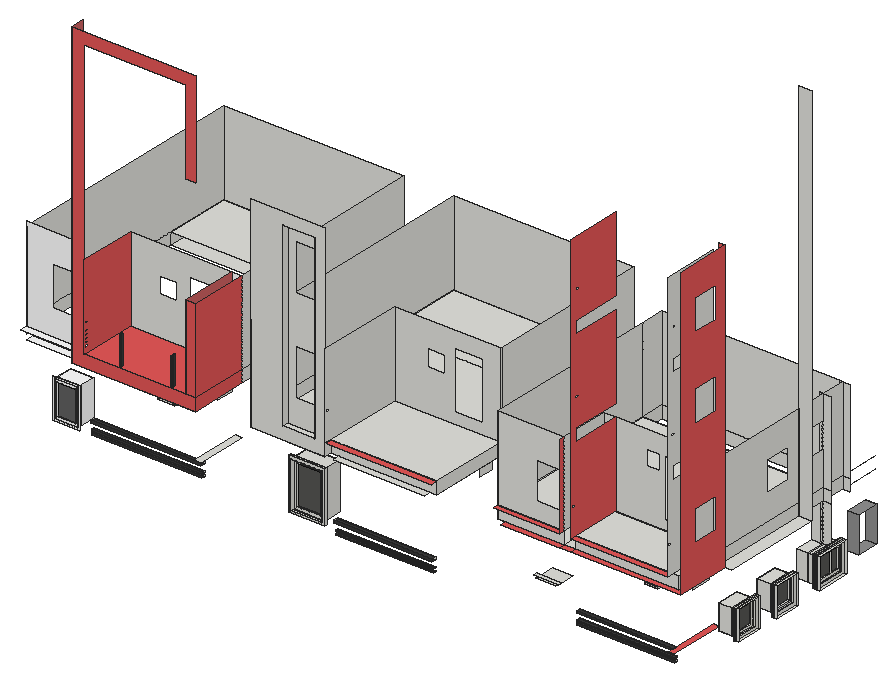
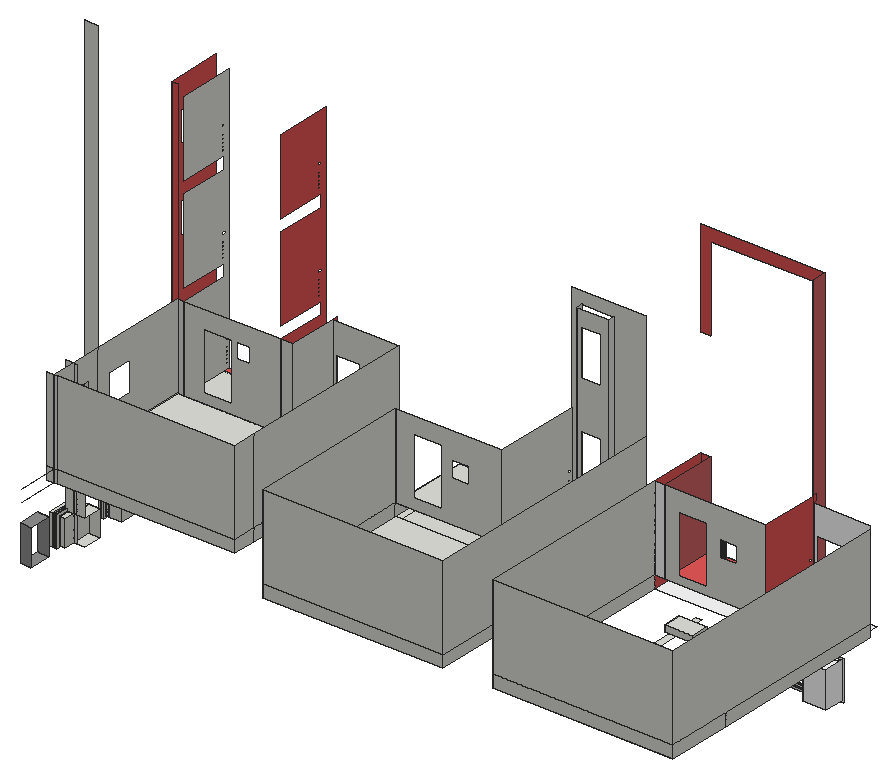
# SketchUp Ruby script. Lengths in inches.
U = 1.inch
M = Sketchup.active_model
def pt(a) = Geom::Point3d.new(a.map { |v| v * U })
def face(e, loops, mat)
  f = e.add_face(loops[0].map { |a| pt(a) })
  loops[1..].each { |l| e.add_face(l.map { |a| pt(a) }).erase! }
  f.material = f.back_material = mat if mat
  f
end
# faces: each face lists its corners as indices into pts; further lists are holes
def faces(e, pts, list, mat = nil) = list.each { |f| face(e, (f[0].is_a?(Array) ? f : [f]).map { |l| l.map { |i| pts[i] } }, mat) }
# xy, xz, yz: faces in a plane at the given z, y or x. An outline is a flat list of corners, or four numbers for a rectangle; further outlines are holes
def ring(l) = l.size == 4 ? [[l[0], l[1]], [l[2], l[1]], [l[2], l[3]], [l[0], l[3]]] : l.each_slice(2).to_a
def flat(e, list, mat, &to3) = list.each { |f| face(e, (f[0].is_a?(Array) ? f : [f]).map { |l| ring(l).map { |u, v| to3.(u, v) } }, mat) }
def xy(e, z, list, mat = nil) = flat(e, list, mat) { |x, y| [x, y, z] }
def xz(e, y, list, mat = nil) = flat(e, list, mat) { |x, z| [x, y, z] }
def yz(e, x, list, mat = nil) = flat(e, list, mat) { |y, z| [x, y, z] }
def lines(e, pts, list) = list.each { |a, b| e.add_line(pt(pts[a]), pt(pts[b])) }
# prism: a flat outline (further loops are holes) pulled along v
def prism(e, loops, v, mat = nil)
  f = face(e, loops, mat); d = Geom::Vector3d.new(v.map { |x| x * U })
  f.pushpull(f.normal.samedirection?(d) ? d.length : -d.length)
end
def box(e, o, s, mat = nil) = prism(e, [[o, [o[0] + s[0], o[1], o[2]], [o[0] + s[0], o[1] + s[1], o[2]], [o[0], o[1] + s[1], o[2]]]], [0, 0, s[2]], mat)
def at(x, y, z, deg = 0) = Geom::Transformation.translation(pt([x, y, z])) * Geom::Transformation.rotation(ORIGIN, Z_AXIS, deg.degrees)
def axes(o, x, y, z) = Geom::Transformation.new([*x, 0, *y, 0, *z, 0, *pt(o).to_a, 1])
def part(name) = M.definitions.add(name)
# library, detail: a bought-in or finely detailed component or shape, given as its bounding box
def library(name, o, s) = part(name).tap { |d| box(d.entities, o, s) }
def detail(e, o, s) = box(e.add_group.entities, o, s)
def put(e, d, t, mat = nil) = e.add_instance(d, t).tap { |i| i.material = mat if mat }
def group(e, t, mat = nil) = e.add_group.tap { |g| g.transformation = t; g.material = mat if mat }.entities
root = M.entities
M.materials.add("Generic").color = [145, 145, 145]
M.materials.add("Generic\#1").color = [206, 99, 99]
M.materials.add("Generic\#2").color = [229, 87, 87]
M.materials.add("[Color M00]").color = [255, 255, 255]
M.materials.add("[Color M07]").color = [58, 58, 58]
M.materials.add("[Translucent Glass Gray]").color = [0, 0, 0]
M.materials["[Translucent Glass Gray]"].alpha = 0.62
M.materials.add("[Translucent Glass Gray]1").color = [128, 128, 128]
M.materials["[Translucent Glass Gray]1"].alpha = 0.5
c1 = part("Group\#5")
xy(c1.entities,0,[[0,0,46.6875,6]],"[Color M00]")
xy(c1.entities,4.48,[[4.48,0,42.2,3]],"[Color M00]")
xy(c1.entities,67.45,[[4.48,0,42.2,3]],"[Color M00]")
xy(c1.entities,71.9375,[[0,0,46.6875,6]],"[Color M00]")
xz(c1.entities,0,[[[0,0,46.6875,71.9375],[4.48,4.48,42.2,67.45]]],"[Color M00]")
xz(c1.entities,3,[[4.48,4.48,42.2,67.45]],"[Translucent Glass Gray]")
xz(c1.entities,6,[[0,0,46.6875,71.9375]],"[Color M00]")
yz(c1.entities,0,[[0,0,6,71.9375]],"[Color M00]")
yz(c1.entities,4.48,[[0,4.48,3,67.45]],"[Color M00]")
yz(c1.entities,42.2,[[0,4.48,3,67.45]],"[Color M00]")
yz(c1.entities,46.6875,[[0,0,6,71.9375]],"[Color M00]")
c2 = part("Group\#9")
xy(c2.entities,0,[[0,0,6,44.5]])
xy(c2.entities,4.64,[[3,4.64,6,39.86]])
xy(c2.entities,45.36,[[3,4.64,6,39.86]])
xy(c2.entities,50,[[0,0,6,44.5]])
xz(c2.entities,0,[[0,0,6,50]])
xz(c2.entities,4.64,[[3,4.64,6,45.36]])
xz(c2.entities,39.86,[[3,4.64,6,45.36]])
xz(c2.entities,44.5,[[0,0,6,50]])
yz(c2.entities,0,[[0,0,44.5,50]])
yz(c2.entities,3,[[4.64,4.64,39.86,45.36]],"[Translucent Glass Gray]")
yz(c2.entities,6,[[[0,0,44.5,50],[4.64,4.64,39.86,45.36]]])
c3 = part("Group\#8")
xy(c3.entities,0,[[0,0,6,59.4375]])
xy(c3.entities,4.64,[[3,4.64,6,54.8]])
xy(c3.entities,46.99,[[3,4.64,6,54.8]])
xy(c3.entities,51.625,[[0,0,6,59.4375]])
xz(c3.entities,0,[[0,0,6,51.625]])
xz(c3.entities,4.64,[[3,4.64,6,46.99]])
xz(c3.entities,54.8,[[3,4.64,6,46.99]])
xz(c3.entities,59.4375,[[0,0,6,51.625]])
yz(c3.entities,0,[[0,0,59.4375,51.625]])
yz(c3.entities,3,[[4.64,4.64,54.8,46.99]],"[Translucent Glass Gray]")
yz(c3.entities,6,[[[0,0,59.4375,51.625],[4.64,4.64,54.8,46.99]]])
c4 = part("Group\#11")
xy(c4.entities,0,[[0,0,27.8125,3]])
xy(c4.entities,27.8125,[[0,0,27.8125,3]])
xz(c4.entities,0,[[0,0,27.8125,27.8125]],"[Translucent Glass Gray]1")
xz(c4.entities,3,[[0,0,27.8125,27.8125]],"[Translucent Glass Gray]1")
yz(c4.entities,0,[[0,0,3,27.8125]])
yz(c4.entities,27.8125,[[0,0,3,27.8125]])
c5 = part("Group\#12")
xy(c5.entities,0,[[0,0,20.25,3]])
xy(c5.entities,24.8125,[[0,0,20.25,3]])
xz(c5.entities,0,[[0,0,20.25,24.8125]],"[Translucent Glass Gray]1")
xz(c5.entities,3,[[0,0,20.25,24.8125]],"[Translucent Glass Gray]1")
yz(c5.entities,0,[[0,0,3,24.8125]])
yz(c5.entities,20.25,[[0,0,3,24.8125]])
xy(root,222.81,[[263.03,103.34,482.8125,108.98]],"[Color M07]")
xy(root,223.99,[[1230.96,102.74,1425.14,108.3]],"[Color M07]")
xy(root,224.3,[[758.59,90.7,954.11,95.51]],"[Color M07]")
xy(root,224.34,[[1452.58,215.23,1457.58,268.54],[1457.58,215.23,1462.21,268.54]])
xy(root,224.91,[[1452.58,310.17,1457.58,363.48],[1457.58,310.17,1462.21,363.48]])
xy(root,226.17,[[758.59,90.7,954.11,95.51]],"[Color M07]")
xy(root,226.18,[[263.03,103.34,482.8125,108.98]],"[Color M07]")
xy(root,226.74,[[1230.96,102.74,1425.14,108.3]],"[Color M07]")
xy(root,227.46,[[1448.58,417.16,1452.58,485.41],[1452.58,417.16,1456.58,485.41],[1456.58,417.16,1462.21,485.41]])
xy(root,228.54,[[192.03,99.8125,238.71,138.75]],"[Color M00]")
xy(root,228.75,[[1419.77,219.63,1452.58,264.13],[1452.58,219.63,1457.58,264.13]])
xy(root,229.28,[[663.18,93.8125,734.35,99.8125]])
xy(root,229.31,[[1419.77,314.57,1452.58,359.07],[1452.58,314.57,1457.58,359.07]])
xy(root,230.06,[[263.03,103.34,482.8125,108.98]],"[Color M07]")
xy(root,230.43,[[1230.96,102.74,1425.14,108.3]],"[Color M07]")
xy(root,230.98,[[758.59,90.7,954.11,95.51]],"[Color M07]")
xy(root,231.86,[[1413.27,421.57,1435.83,459.8125],[1435.83,421.57,1448.58,459.8125],[1448.58,421.57,1452.58,481],[1452.58,421.57,1456.58,481],[1435.83,459.8125,1448.58,481]])
xy(root,232.86,[[758.59,90.7,954.11,95.51]],"[Color M07]")
xy(root,233.18,[[1230.96,102.74,1425.14,108.3]],"[Color M07]")
xy(root,233.43,[[263.03,103.34,482.8125,108.98]],"[Color M07]")
xy(root,233.65,[[667.55,93.8125,729.98,99.8125],[667.55,99.8125,729.98,137.6875]])
xy(root,239.12,[[1429.21,528.77,1451.02,572.96]],"Generic")
xy(root,245.06,[[443.78,103.76,445.34,107.89],[446.53,103.76,448.09,107.89]])
xy(root,245.06,[[[263.03,100.96,482.8125,108.98],[443.78,103.76,445.34,107.89],[446.53,103.76,448.09,107.89]]],"[Color M07]")
xy(root,245.43,[[1230.96,100.55,1425.14,108.3]],"[Color M07]")
xy(root,245.62,[[333.84,103.76,335.4,107.89]])
xy(root,245.73,[[758.59,87.57,954.11,95.51]],"[Color M07]")
xy(root,245.93,[[336.59,103.76,338.15,107.89]])
xy(root,249.99,[[263.03,100.96,482.8125,108.98]],"[Color M07]")
xy(root,250.36,[[1425.14,88,1435.83,199.25]],"Generic\#2")
xy(root,250.36,[[1230.96,100.55,1425.14,108.3]],"[Color M07]")
xy(root,251.17,[[758.59,87.57,954.11,95.51]],"[Color M07]")
xy(root,262.625,[[482.8125,84.5,495.5,187.125]])
xy(root,275.46,[[808.05,253.75,841.375,258.8125]])
xy(root,275.88,[[331.98,182.0625,365.3125,187.125]])
xy(root,278.22,[[810.81,253.75,838.62,258.8125],[810.81,258.8125,838.62,292.8125]])
xy(root,278.6,[[1292.01,194.1875,1317.77,199.25]])
xy(root,278.63,[[334.74,182.0625,362.55,187.125],[334.74,187.125,362.55,221.125]])
xy(root,278.75,[[1419.77,219.63,1452.58,264.13],[1452.58,219.63,1457.58,264.13]])
xy(root,279.31,[[1419.77,314.57,1452.58,359.07],[1452.58,314.57,1457.58,359.07]])
xy(root,281.36,[[1294.76,194.1875,1315.01,199.25],[1294.76,199.25,1315.01,212.4375]])
xy(root,283.15,[[1452.58,215.23,1457.58,268.54],[1457.58,215.23,1462.21,268.54]])
xy(root,283.49,[[1413.27,421.57,1435.83,459.8125],[1435.83,421.57,1448.58,459.8125],[1448.58,421.57,1452.58,481],[1452.58,421.57,1456.58,481],[1435.83,459.8125,1448.58,481]])
xy(root,283.71,[[1452.58,310.17,1457.58,363.48],[1457.58,310.17,1462.21,363.48]])
xy(root,284.75,[[1156.27,93.8125,1196.2,99.8125],[1156.27,99.8125,1196.2,134.3125]])
xy(root,287.89,[[1448.58,417.16,1452.58,485.41],[1452.58,417.16,1456.58,485.41],[1456.58,417.16,1462.21,485.41]])
xy(root,289.12,[[1151.9,93.8125,1200.57,99.8125]])
xy(root,300.48,[[192.03,99.8125,238.71,138.75]],"[Color M00]")
xy(root,306.03,[[810.81,253.75,838.62,258.8125],[810.81,258.8125,838.62,292.8125]])
xy(root,306.17,[[1294.76,194.1875,1315.01,199.25],[1294.76,199.25,1315.01,212.4375]])
xy(root,306.45,[[334.74,182.0625,362.55,187.125],[334.74,187.125,362.55,221.125]])
xy(root,308.79,[[808.05,253.75,841.375,258.8125]])
xy(root,308.93,[[1292.01,194.1875,1317.77,199.25]])
xy(root,309.2,[[331.98,182.0625,365.3125,187.125]])
xy(root,310.62,[[1429.21,528.77,1451.02,572.96]],"Generic")
xy(root,314.12,[[1327.46,199.25,1383.27,240]])
xy(root,321.51,[[856.48,258.8125,912.29,288.3125]])
xy(root,326.71,[[667.55,93.8125,729.98,99.8125],[667.55,99.8125,729.98,137.6875]])
xy(root,327.08,[[392.26,187.125,448.07,220.9375]])
xy(root,331.08,[[663.18,93.8125,734.35,99.8125]])
xy(root,360,[[594.11,86,741.96,99.8125],[758.59,86,940.8,99.8125],[594.11,99.8125,594.11,459.8125,954.11,459.8125,954.11,258.8125,741.96,258.8125,741.96,99.8125],[741.96,99.8125,758.59,258.8125],[758.59,99.8125,940.8,258.8125],
  [940.8,99.8125,954.11,258.8125],[1075.83,99.8125,1075.83,459.8125,1413.27,459.8125,1413.27,199.25,1207.39,199.25,1207.39,99.8125],[1207.39,99.8125,1230.96,199.25],[1413.27,199.25,1435.83,398.12],[1435.83,199.25,1462.21,398.12],
  [1413.27,398.12,1435.83,459.8125],[135.5,459.8125,495.5,590.625],[594.11,459.8125,954.11,590.625]])
xy(root,360,[[1091.08,88,1207.39,99.8125],[1207.39,88,1230.96,99.8125],[1230.96,88,1230.96,99.8125,1435.83,99.8125,1435.83,199.25,1448.83,199.25,1448.83,88],[1230.96,99.8125,1435.83,199.25]],"Generic\#2")
xy(root,360,[[248.28,71.5,248.28,84.5,147.6875,84.5,147.6875,99.8125,263.03,99.8125,263.03,187.125,495.5,187.125,495.5,71.5]],"[Color M00]")
xy(root,373.375,[[135.5,84.5,248.28,99.8125]],"[Color M00]")
xy(root,384,[[339.06,76.97,340.62,80.4375],[341.81,76.97,343.37,80.4375],[442.43,76.97,444,80.4375],[445.18,76.97,446.75,80.4375],[657.35,86,720.59,99.8125],
  [741.96,99.8125,954.11,258.8125],[1075.83,99.8125,1075.83,459.8125,1435.83,459.8125,1435.83,199.25,1207.39,199.25,1207.39,99.8125],[1230.96,99.8125,1423.39,199.25],[1423.39,99.8125,1435.83,199.25],[135.5,459.8125,495.5,590.625],
  [594.11,459.8125,954.11,590.625]])
xy(root,384,[[[272.78,71.5,475.8125,187.125],[445.18,76.97,446.75,80.4375],[442.43,76.97,444,80.4375],[341.81,76.97,343.37,80.4375],[339.06,76.97,340.62,80.4375]],[741.96,86,954.11,99.8125],[1075.83,88,1207.39,99.8125],[1230.96,88,1423.39,99.8125]],"Generic\#2")
xy(root,384,[[475.8125,71.5,495.5,187.125]],"[Color M00]")
xz(root,71.5,[[248.28,360,495.5,360,495.5,384,272.78,384,272.78,936,475.8125,936,475.8125,768,495.5,768,495.5,960,248.28,960],[475.8125,384,495.5,552]],"Generic\#2")
xz(root,76.97,[[339.06,384,340.62,441.31],[341.81,384,343.37,441.31],[442.43,384,444,438.37],[445.18,384,446.75,441.06]],"[Color M07]")
xz(root,80.4375,[[339.06,384,340.62,394.36],[341.81,384,343.37,394.36],[445.18,384,446.75,394.36]])
xz(root,86,[[[594.11,360,741.96,768],[657.35,384,720.59,744]]])
xz(root,87.57,[[758.59,245.73,954.11,251.17]],"[Color M07]")
xz(root,90.7,[[758.59,224.3,954.11,226.17],[758.59,230.98,954.11,232.86]],"[Color M07]")
xz(root,93.8125,[[[663.18,229.28,734.35,331.08],[667.55,233.65,729.98,326.71]]])
xz(root,95.51,[[758.59,224.3,954.11,226.17],[758.59,230.98,954.11,232.86],[758.59,245.73,954.11,251.17]])
xz(root,99.8125,[[[663.18,229.28,734.35,331.08],[667.55,233.65,729.98,326.71]],[741.96,360,954.11,384],[1075.83,360,1207.39,384],[1230.96,360,1435.83,384],[[657.35,384,720.59,744],[672.35,621.05,712.33,713.66],[672.35,433.8,712.33,526.41]],
  [[1075.83,384,1207.39,552],[1151.9,418.07,1200.57,491.43]]])
xz(root,99.8125,[[[188.42,224.94,242.3125,304.08],[192.03,228.54,238.71,300.48]],[[135.5,373.375,248.28,560.8125],[188.42,424.75,242.3125,503.89]]],"[Color M00]")
xz(root,100.55,[[1230.96,245.43,1425.14,250.36]],"[Color M07]")
xz(root,100.96,[[263.03,245.06,482.8125,249.99]],"[Color M07]")
xz(root,102.74,[[1230.96,223.99,1425.14,226.74],[1230.96,230.43,1425.14,233.18]],"[Color M07]")
xz(root,103.34,[[263.03,222.81,482.8125,226.18],[263.03,230.06,482.8125,233.43]],"[Color M07]")
xz(root,108.3,[[1230.96,223.99,1425.14,226.74],[1230.96,230.43,1425.14,233.18],[1230.96,245.43,1425.14,250.36]])
xz(root,108.98,[[263.03,222.81,482.8125,226.18],[263.03,230.06,482.8125,233.43],[263.03,245.06,482.8125,249.99]])
xz(root,137.6875,[[667.55,233.65,729.98,326.71]])
xz(root,138.75,[[192.03,228.54,238.71,300.48]],"[Color M00]")
xz(root,182.0625,[[[331.98,275.88,365.3125,309.2],[334.74,278.63,362.55,306.45]]])
xz(root,187.125,[[[331.98,275.88,365.3125,309.2],[334.74,278.63,362.55,306.45]],[[272.78,384,475.8125,552],[392.26,399.1875,448.07,512.73],[331.98,461.13,365.3125,494.45]]])
xz(root,187.125,[[475.8125,384,495.5,552]],"[Color M00]")
xz(root,194.1875,[[[1292.01,278.6,1317.77,308.93],[1294.76,281.36,1315.01,306.17]]])
xz(root,199.25,[[[1292.01,278.6,1317.77,308.93],[1294.76,281.36,1315.01,306.17]],[1207.39,384,1230.96,552],[[1230.96,384,1423.39,552],[1327.46,403.35,1383.27,516.9],[1292.01,486.72,1317.77,517.05]],[1423.39,384,1435.83,552]])
xz(root,199.25,[[1435.83,360,1448.83,936]],"Generic\#2")
xz(root,212.4375,[[1294.76,281.36,1315.01,306.17]])
xz(root,215.23,[[1452.58,224.34,1457.58,283.15],[1457.58,224.34,1462.21,283.15]])
xz(root,219.63,[[1419.77,228.75,1452.58,278.75],[1452.58,228.75,1457.58,278.75]])
xz(root,220.9375,[[392.26,313.66,448.07,327.08]])
xz(root,221.125,[[334.74,278.63,362.55,306.45]])
xz(root,240,[[1327.46,297.87,1383.27,314.12]])
xz(root,253.75,[[[808.05,275.46,841.375,308.79],[810.81,278.22,838.62,306.03]]])
xz(root,258.8125,[[[808.05,275.46,841.375,308.79],[810.81,278.22,838.62,306.03]],[[741.96,384,954.11,552],[862.05,405.73,917.86,519.27],[808.05,467.09,841.375,500.42]]])
xz(root,264.13,[[1419.77,228.75,1452.58,278.75],[1452.58,228.75,1457.58,278.75]])
xz(root,268.54,[[1452.58,224.34,1457.58,283.15],[1457.58,224.34,1462.21,283.15]])
xz(root,288.3125,[[856.48,307.2,912.29,321.51]])
xz(root,292.8125,[[810.81,278.22,838.62,306.03]])
xz(root,310.17,[[1452.58,224.91,1457.58,283.71],[1457.58,224.91,1462.21,283.71]])
xz(root,314.57,[[1419.77,229.31,1452.58,279.31],[1452.58,229.31,1457.58,279.31]])
xz(root,359.07,[[1419.77,229.31,1452.58,279.31],[1452.58,229.31,1457.58,279.31]])
xz(root,363.48,[[1452.58,224.91,1457.58,283.71],[1457.58,224.91,1462.21,283.71]])
xz(root,398.12,[[1435.83,360,1462.21,1128]])
xz(root,417.16,[[1448.58,227.46,1452.58,287.89],[1452.58,227.46,1456.58,287.89],[1456.58,227.46,1462.21,287.89]])
xz(root,421.57,[[1413.27,231.86,1435.83,283.49],[1435.83,231.86,1448.58,283.49],[1448.58,231.86,1452.58,283.49],[1452.58,231.86,1456.58,283.49]])
xz(root,459.8125,[[1429.21,231.86,1433.58,283.49],[1433.58,231.86,1435.83,283.49],[1435.83,231.86,1451.02,283.49],[1413.27,283.49,1429.21,360],[1429.21,283.49,1433.58,360],
  [1433.58,283.49,1435.83,360],[1435.83,283.49,1451.02,360],[1075.83,360,1429.21,384],[1429.21,360,1433.58,384],[1433.58,360,1435.83,384],
  [1435.83,360,1451.02,384],[1429.21,384,1433.58,552],[1433.58,384,1435.83,552],[1435.83,384,1451.02,552]])
xz(root,481,[[1435.83,231.86,1448.58,283.49],[1448.58,231.86,1452.58,283.49],[1452.58,231.86,1456.58,283.49]])
xz(root,485.41,[[1448.58,227.46,1452.58,287.89],[1452.58,227.46,1456.58,287.89],[1456.58,227.46,1462.21,287.89]])
xz(root,507.75,[[1075.83,360,1429.21,384],[1429.21,360,1435.83,384],[1435.83,360,1451.02,384],[1075.83,384,1429.21,552],[1429.21,384,1435.83,552],
  [1435.83,384,1451.02,552]])
xz(root,528.77,[[1429.21,239.12,1451.02,310.62]],"Generic")
xz(root,572.96,[[1429.21,239.12,1451.02,310.62]],"Generic")
xz(root,590.625,[[135.5,360,495.5,384],[594.11,360,954.11,384],[135.5,384,495.5,552],[594.11,384,954.11,552]])
yz(root,135.5,[[99.8125,360,459.8125,384],[459.8125,360,590.625,384],[99.8125,384,590.625,552]])
yz(root,192.03,[[99.8125,228.54,138.75,300.48]],"[Color M00]")
yz(root,238.71,[[99.8125,228.54,138.75,300.48]],"[Color M00]")
yz(root,248.28,[[71.5,360,71.5,960,99.8125,960,99.8125,576,90.625,576,90.625,560.8125,99.8125,560.8125,99.8125,373.375,84.5,373.375,84.5,360]],"Generic\#1")
yz(root,263.03,[[103.34,222.81,108.98,226.18],[103.34,230.06,108.98,233.43],[100.96,245.06,108.98,249.99]])
yz(root,272.78,[[[71.5,384,77.61,384,77.61,394.36,74.79,394.36,74.79,397.74,80.4375,397.74,80.4375,394.36,77.61,394.36,77.61,384,187.125,384,187.125,552,71.5,552],[72.41,437.31,80.4375,442.24],[74.79,401.61,80.4375,404.99],[74.79,408.18,80.4375,411.55],[74.79,415.24,80.4375,418.62],[74.79,422.31,80.4375,425.68]]],"Generic\#2")
yz(root,331.98,[[182.0625,275.88,187.125,309.2]])
yz(root,334.74,[[182.0625,278.63,187.125,306.45],[187.125,278.63,221.125,306.45]])
yz(root,339.06,[[76.97,384,80.4375,441.31]],"[Color M07]")
yz(root,340.62,[[76.97,384,80.4375,441.31]],"[Color M07]")
yz(root,341.81,[[76.97,384,80.4375,441.31]],"[Color M07]")
yz(root,343.37,[[76.97,384,80.4375,441.31]],"[Color M07]")
yz(root,362.55,[[182.0625,278.63,187.125,306.45],[187.125,278.63,221.125,306.45]])
yz(root,365.3125,[[182.0625,275.88,187.125,309.2]])
yz(root,392.26,[[187.125,313.66,220.9375,327.08]])
yz(root,442.43,[[76.97,384,80.4375,438.37]],"[Color M07]")
yz(root,444,[[76.97,384,80.4375,438.37]],"[Color M07]")
yz(root,445.18,[[76.97,384,80.4375,441.06]],"[Color M07]")
yz(root,446.75,[[76.97,384,80.4375,441.06]],"[Color M07]")
yz(root,448.07,[[187.125,313.66,220.9375,327.08]])
yz(root,475.8125,[[71.5,384,187.125,552]],"Generic\#1")
yz(root,495.5,[[187.125,360,590.625,384],[187.125,384,590.625,552]])
yz(root,495.5,[[71.5,360,187.125,384],[71.5,384,187.125,552]],"Generic\#2")
yz(root,594.11,[[86,360,459.8125,384],[459.8125,360,590.625,384],[86,384,590.625,552]])
yz(root,657.35,[[86,384,99.8125,744]])
yz(root,663.18,[[93.8125,229.28,99.8125,331.08]])
yz(root,667.55,[[93.8125,233.65,99.8125,326.71],[99.8125,233.65,137.6875,326.71]])
yz(root,720.59,[[86,384,99.8125,744]])
yz(root,729.98,[[93.8125,233.65,99.8125,326.71],[99.8125,233.65,137.6875,326.71]])
yz(root,734.35,[[93.8125,229.28,99.8125,331.08]])
yz(root,741.96,[[86,360,99.8125,384],[[86,384,258.8125,552],[87.39,437.85,95.33,443.28],[90.52,395.27,95.33,397.15],[90.27,401.9,95.08,403.77],[90.33,408.77,95.14,410.65],[90.27,416.28,95.08,418.16],[90.39,422.85,95.2,424.72]]])
yz(root,758.59,[[90.7,224.3,95.51,226.17],[90.7,230.98,95.51,232.86],[87.57,245.73,95.51,251.17]])
yz(root,808.05,[[253.75,275.46,258.8125,308.79]])
yz(root,810.81,[[253.75,278.22,258.8125,306.03],[258.8125,278.22,292.8125,306.03]])
yz(root,838.62,[[253.75,278.22,258.8125,306.03],[258.8125,278.22,292.8125,306.03]])
yz(root,841.375,[[253.75,275.46,258.8125,308.79]])
yz(root,856.48,[[258.8125,307.2,288.3125,321.51]])
yz(root,912.29,[[258.8125,307.2,288.3125,321.51]])
yz(root,954.11,[[99.8125,360,260.5,384],[260.5,360,590.625,384],[258.8125,384,260.5,552],[260.5,384,590.625,552]])
yz(root,1075.83,[[99.8125,360,459.8125,384],[459.8125,360,507.75,384],[99.8125,384,459.8125,552],[459.8125,384,507.75,552]])
yz(root,1207.39,[[99.8125,384,199.25,552]])
yz(root,1207.39,[[88,384,99.8125,552]],"Generic\#2")
yz(root,1230.96,[[102.74,223.99,108.3,226.74],[102.74,230.43,108.3,233.18],[100.55,245.43,108.3,250.36]])
yz(root,1230.96,[[[88,384,199.25,384,199.25,552,99.8125,552,99.8125,576,199.25,576,199.25,744,99.8125,744,99.8125,768,199.25,768,199.25,917.875,88,917.875],[96.68,629.37,106.62,634.31],[88.89,437.21,96.64,442.14],[99.8125,821.5625,106.62,826.5],[101.06,778.5,106.62,781.25],[101.06,785.4375,106.62,788.1875],[101.06,792.4375,106.62,795.1875],[101.06,799.6875,106.62,802.4375],[101.06,806.5625,106.62,809.3125],[101.06,614.37,106.62,617.12],[101.06,607.25,106.62,610],[101.06,600.625,106.62,603.375],[101.06,593.5625,106.62,596.3125],[91.08,422.82,96.64,425.57],[91.08,415.32,96.64,418.07],[91.08,408.7,96.64,411.45],[91.08,401.51,96.64,404.26],[91.08,394.51,96.64,397.26],[101.06,586.3125,106.62,589.0625]]],"Generic\#2")
yz(root,1292.01,[[194.1875,278.6,199.25,308.93]])
yz(root,1294.76,[[194.1875,281.36,199.25,306.17],[199.25,281.36,212.4375,306.17]])
yz(root,1315.01,[[194.1875,281.36,199.25,306.17],[199.25,281.36,212.4375,306.17]])
yz(root,1317.77,[[194.1875,278.6,199.25,308.93]])
yz(root,1327.46,[[199.25,297.87,240,314.12]])
yz(root,1383.27,[[199.25,297.87,240,314.12]])
yz(root,1419.77,[[219.63,228.75,264.13,278.75],[314.57,229.31,359.07,279.31]])
yz(root,1423.39,[[[88,384,88,917.875,199.25,917.875,199.25,768,99.8125,768,99.8125,744,199.25,744,199.25,576,99.8125,576,99.8125,552,199.25,552,199.25,384],[96.68,629.37,106.62,634.31],[88.89,437.21,96.64,442.14],[99.8125,821.5625,106.62,826.5],[101.06,806.5625,106.62,809.3125],[101.06,799.6875,106.62,802.4375],[101.06,792.4375,106.62,795.1875],[101.06,785.4375,106.62,788.1875],[101.06,778.5,106.62,781.25],[101.06,614.37,106.62,617.12],[101.06,607.25,106.62,610],[101.06,600.625,106.62,603.375],[101.06,593.5625,106.62,596.3125],[101.06,586.3125,106.62,589.0625],[91.08,422.82,96.64,425.57],[91.08,415.32,96.64,418.07],[91.08,408.7,96.64,411.45],[91.08,401.51,96.64,404.26],[91.08,394.51,96.64,397.26]]])
yz(root,1425.14,[[100.55,245.43,108.3,250.36]])
yz(root,1435.83,[[421.57,231.86,459.8125,283.49],[459.8125,231.86,481,283.49],[99.8125,360,199.25,384],[199.25,360,398.12,384],[398.12,360,459.8125,384],
  [459.8125,360,507.75,384],[[199.25,384,398.12,552],[318.51,437.21,371.82,496.01]],[398.12,384,398.12,552,459.8125,552,459.8125,503.36,421.57,503.36,421.57,451.74,459.8125,451.74,459.8125,384],[459.8125,384,507.75,384,507.75,552,459.8125,552,459.8125,503.36,481,503.36,481,451.74,459.8125,451.74]])
yz(root,1448.58,[[[417.16,227.46,485.41,287.89],[421.57,231.86,481,283.49]]])
yz(root,1448.83,[[[88,360,199.25,936],[123.62,813.55,175.61,875.42],[123.62,650.36,175.61,712.23],[123.62,437.05,175.61,498.92]]],"Generic\#2")
yz(root,1452.58,[[[215.23,224.34,268.54,283.15],[219.63,228.75,264.13,278.75]],[[310.17,224.91,363.48,283.71],[314.57,229.31,359.07,279.31]],[[417.16,227.46,485.41,287.89],[421.57,231.86,481,283.49]]])
yz(root,1456.58,[[[417.16,227.46,485.41,287.89],[421.57,231.86,481,283.49]]])
yz(root,1457.58,[[[215.23,224.34,268.54,283.15],[219.63,228.75,264.13,278.75]],[[310.17,224.91,363.48,283.71],[314.57,229.31,359.07,279.31]]])
p = [[263.03,105.8125,225],[482.8125,105.8125,225],[263.03,105.8125,232],[482.8125,105.8125,232],[333.84,103.76,245.62],[333.84,103.76,249.99],
  [335.4,103.76,245.62],[335.4,103.76,249.99],[333.84,107.89,245.62],[333.84,107.89,249.99],[335.4,107.89,245.62],[335.4,107.89,249.99],
  [336.59,103.76,245.93],[336.59,103.76,249.99],[338.15,103.76,245.93],[338.15,103.76,249.99],[336.59,107.89,245.93],[336.59,107.89,249.99],
  [338.15,107.89,245.93],[338.15,107.89,249.99],[443.78,103.76,245.06],[443.78,103.76,249.99],[445.34,103.76,245.06],[445.34,103.76,249.99],
  [443.78,107.89,245.06],[443.78,107.89,249.99],[445.34,107.89,245.06],[445.34,107.89,249.99],[446.53,103.76,245.06],[446.53,103.76,249.99],
  [448.09,103.76,245.06],[448.09,103.76,249.99],[446.53,107.89,245.06],[446.53,107.89,249.99],[448.09,107.89,245.06],[448.09,107.89,249.99],
  [1435.83,507.75,384],[1435.83,590.625,384],[1435.83,507.75,360],[1435.83,590.625,360],[758.59,92.91,225],[940.8,92.91,225],
  [758.59,92.91,232],[940.8,92.91,232],[758.59,92.91,247],[940.8,92.91,247],[1230.96,105,225],[1425.14,105,225],
  [1230.96,105,232],[1425.14,105,232],[1230.96,105,247],[1425.14,105,247]]
lines(root,p,[[0,1],[2,3],[4,5],[6,7],[8,9],[10,11],[12,13],[14,15],[16,17],[18,19],[20,21],[22,23],
  [24,25],[26,27],[28,29],[30,31],[32,33],[34,35],[36,37],[38,39],[40,41],[42,43],[44,45],[46,47],
  [48,49],[50,51]])
put(root,c1,at(192.03,99.8125,228.6))
put(root,c2,at(1446.58,219.63,228.75))
put(root,c2,at(1446.58,314.57,229.31))
put(root,c3,at(1446.58,421.57,231.86))
g1 = group(root,at(667.55,99.8125,233.65))
xy(g1,0,[[0,0,62.4375,6]])
xy(g1,7.24,[[7.24,0,55.19,3]])
xy(g1,85.82,[[7.24,0,55.19,3]])
xy(g1,93.0625,[[0,0,62.4375,6]])
xz(g1,0,[[[0,0,62.4375,93.0625],[7.24,7.24,55.19,85.82]]])
xz(g1,3,[[7.24,7.24,55.19,85.82]],"[Translucent Glass Gray]")
xz(g1,6,[[0,0,62.4375,93.0625]])
yz(g1,0,[[0,0,6,93.0625]])
yz(g1,7.24,[[0,7.24,3,85.82]])
yz(g1,55.19,[[0,7.24,3,85.82]])
yz(g1,62.4375,[[0,0,6,93.0625]])
put(root,c4,at(810.81,258.8125,278.22))
put(root,c4,at(334.74,187.125,278.63))
put(root,c5,at(1294.76,199.25,281.36))
